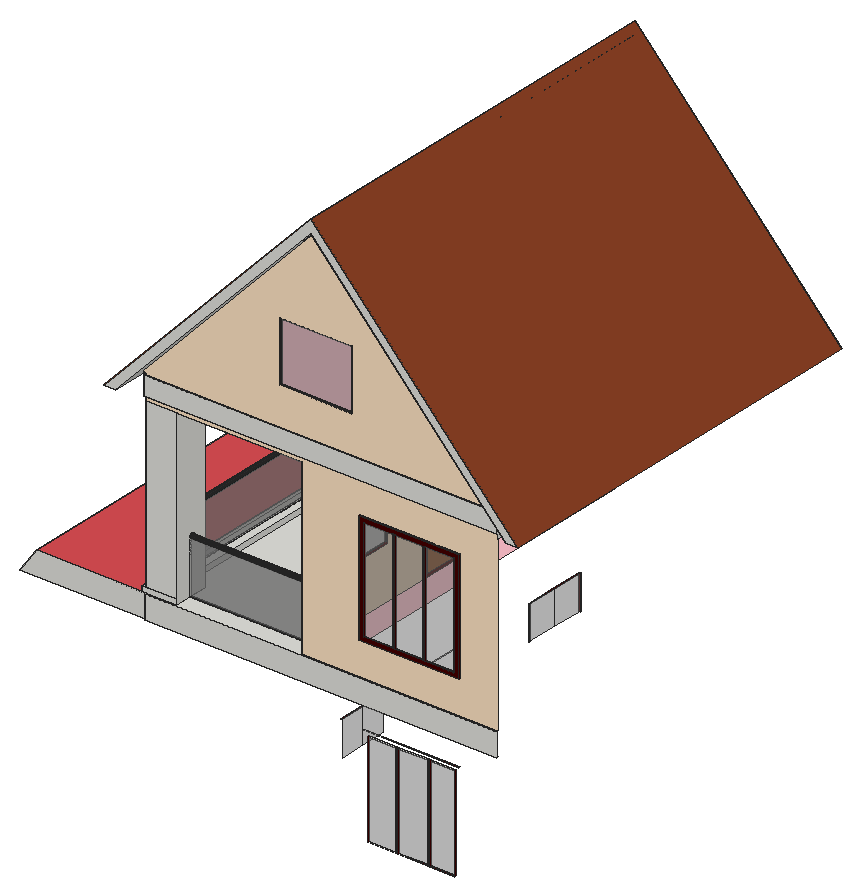
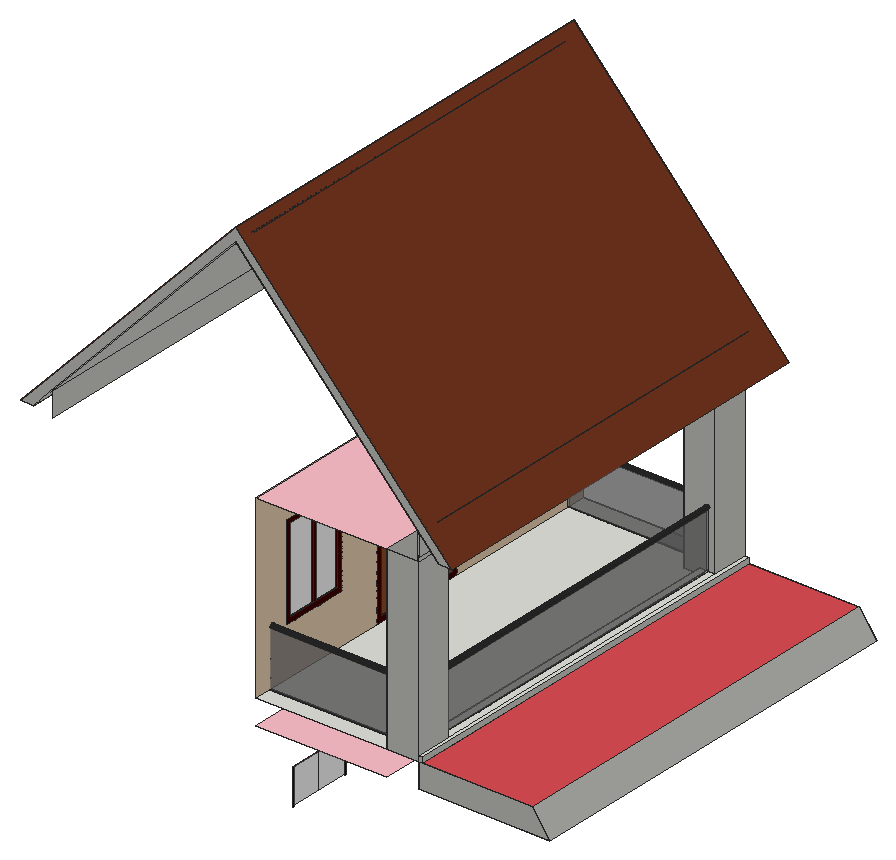
# SketchUp Ruby script. Lengths in inches.
U = 1.inch
M = Sketchup.active_model
def pt(a) = Geom::Point3d.new(a.map { |v| v * U })
def face(e, loops, mat)
  f = e.add_face(loops[0].map { |a| pt(a) })
  loops[1..].each { |l| e.add_face(l.map { |a| pt(a) }).erase! }
  f.material = f.back_material = mat if mat
  f
end
# faces: each face lists its corners as indices into pts; further lists are holes
def faces(e, pts, list, mat = nil) = list.each { |f| face(e, (f[0].is_a?(Array) ? f : [f]).map { |l| l.map { |i| pts[i] } }, mat) }
# xy, xz, yz: faces in a plane at the given z, y or x. An outline is a flat list of corners, or four numbers for a rectangle; further outlines are holes
def ring(l) = l.size == 4 ? [[l[0], l[1]], [l[2], l[1]], [l[2], l[3]], [l[0], l[3]]] : l.each_slice(2).to_a
def flat(e, list, mat, &to3) = list.each { |f| face(e, (f[0].is_a?(Array) ? f : [f]).map { |l| ring(l).map { |u, v| to3.(u, v) } }, mat) }
def xy(e, z, list, mat = nil) = flat(e, list, mat) { |x, y| [x, y, z] }
def xz(e, y, list, mat = nil) = flat(e, list, mat) { |x, z| [x, y, z] }
def yz(e, x, list, mat = nil) = flat(e, list, mat) { |y, z| [x, y, z] }
def lines(e, pts, list) = list.each { |a, b| e.add_line(pt(pts[a]), pt(pts[b])) }
# prism: a flat outline (further loops are holes) pulled along v
def prism(e, loops, v, mat = nil)
  f = face(e, loops, mat); d = Geom::Vector3d.new(v.map { |x| x * U })
  f.pushpull(f.normal.samedirection?(d) ? d.length : -d.length)
end
def box(e, o, s, mat = nil) = prism(e, [[o, [o[0] + s[0], o[1], o[2]], [o[0] + s[0], o[1] + s[1], o[2]], [o[0], o[1] + s[1], o[2]]]], [0, 0, s[2]], mat)
def at(x, y, z, deg = 0) = Geom::Transformation.translation(pt([x, y, z])) * Geom::Transformation.rotation(ORIGIN, Z_AXIS, deg.degrees)
def axes(o, x, y, z) = Geom::Transformation.new([*x, 0, *y, 0, *z, 0, *pt(o).to_a, 1])
def part(name) = M.definitions.add(name)
# library, detail: a bought-in or finely detailed component or shape, given as its bounding box
def library(name, o, s) = part(name).tap { |d| box(d.entities, o, s) }
def detail(e, o, s) = box(e.add_group.entities, o, s)
def put(e, d, t, mat = nil) = e.add_instance(d, t).tap { |i| i.material = mat if mat }
def group(e, t, mat = nil) = e.add_group.tap { |g| g.transformation = t; g.material = mat if mat }.entities
root = M.entities
M.materials.add("[0006_Pink]").color = [255, 192, 203]
M.materials.add("[0012_Bisque]").color = [255, 228, 196]
M.materials.add("[0022_Maroon]").color = [68, 0, 0]
M.materials.add("[0137_Black]").color = [45, 45, 45]
M.materials.add("[Roofing Scalloped Ornate]").color = [219, 78, 83]
M.materials.add("[Roofing Tile Spanish]").color = [138, 64, 36]
M.materials.add("[Translucent Glass Gray]").color = [128, 128, 128]
M.materials["[Translucent Glass Gray]"].alpha = 0.5
M.materials.add("[Wood Cherry Original]").color = [152, 86, 42]
xy(root,126.66,[[577.0625,82,581.0625,84],[625.98,82,629.98,84]])
xy(root,126.66,[[535.0625,82,577.0625,84],[581.0625,82,625.98,84],[629.98,82,667.98,84]],"[0022_Maroon]")
xy(root,140.25,[[432,383.84,434,385.71],[432,397.59,434,399.46]])
xy(root,163.32,[[432,383.84,434,385.71],[432,397.59,434,399.46]])
xy(root,226.5,[[432,159.23,434,238.92],[432,518.52,434,566.6875],[432,566.6875,434,614.85]],"[0022_Maroon]")
xy(root,227.44,[[432,334.98,434,391.49],[432,391.49,434,447.99]])
xy(root,271.7,[[535.0625,82,577.0625,84],[577.0625,82,581.0625,84],[581.0625,82,625.98,84],[625.98,82,629.98,84],[629.98,82,667.98,84]])
xy(root,278.46,[[528.3,82,674.74,84]],"[0022_Maroon]")
xy(root,312,[[432,82,732,84]])
xy(root,312,[[193.3125,82,193.3125,84,240,84,240,138.5625,193.3125,138.5625,193.3125,629.4375,240,629.4375,240,684,432,684,432,82],[0,84,193.3125,684]],"[0006_Pink]")
xy(root,348,[[193.3125,82,432,82,432,109.28,240,109.28,240,84,193.3125,84],[432,82,732,84],[187.3125,84,193.3125,138.5625],[193.3125,84,240,138.5625],[240,109.28,432,111.28],
  [240,111.28,432,111.28,432,656.72,240,656.72,240,629.4375,216.66,629.4375,216.66,138.5625,240,138.5625],[187.3125,138.5625,193.3125,629.4375],[193.3125,138.5625,216.66,629.4375],[187.3125,629.4375,193.3125,684],[193.3125,629.4375,240,684],
  [240,656.72,432,658.72],[240,658.72,432,684]])
xy(root,348,[[25.13,84,187.3125,684]],"[Roofing Scalloped Ornate]")
xy(root,355.14,[[432,322.1875,434,389.08],[432,389.08,434,455.96]],"[0022_Maroon]")
xy(root,356,[[187.3125,84,193.3125,684],[193.3125,138.5625,202.98,629.4375],[202.98,138.5625,204.98,629.4375],[204.98,138.5625,216.66,629.4375]])
xy(root,399.1,[[521.24,82,673.49,84]])
xy(root,406.125,[[572.26,82,576.26,84],[618.46,82,622.46,84]])
xy(root,406.125,[[528.26,82,572.26,84],[576.26,82,618.46,84],[622.46,82,666.46,84]],"[0022_Maroon]")
xy(root,427.0625,[[432,534.59,434,574.62],[432,578.62,434,622.65]],"[0022_Maroon]")
xy(root,429,[[240,109.28,432,111.28],[240,656.72,432,658.72]])
xy(root,432.76,[[432,157.6,434,195.91],[432,199.91,434,242.21]],"[0022_Maroon]")
xy(root,437,[[202.98,138.5625,204.98,629.4375]])
xy(root,447.4,[[432,378.54,434,380.85],[432,395.92,434,398.23]])
xy(root,473.15,[[432,378.54,434,380.85],[432,395.92,434,398.23]])
xy(root,551.5,[[432,157.6,434,195.91],[432,199.91,434,242.21],[432,534.59,434,574.62],[432,578.62,434,622.65]],"[0022_Maroon]")
xy(root,551.61,[[432,389.08,434,455.96]])
xy(root,551.61,[[432,322.1875,434,389.08]],"[0022_Maroon]")
xy(root,563.02,[[572.26,82,576.26,84],[618.46,82,622.46,84]])
xy(root,563.02,[[528.26,82,572.26,84],[576.26,82,618.46,84],[622.46,82,666.46,84]],"[0022_Maroon]")
xy(root,570.04,[[521.24,82,673.49,84]],"[0022_Maroon]")
xy(root,612,[[240,84,240,138.5625,193.3125,138.5625,193.3125,629.4375,240,629.4375,240,684,432,684,432,84]],"[0006_Pink]")
xy(root,619.2,[[191.3125,82,732,84],[191.3125,84,193.3125,684]])
xy(root,621.68,[[141.01,68.125,160.14,688.3125],[756.56,68.125,775.69,688.3125]])
xy(root,648,[[191.3125,82,732,84],[191.3125,84,193.3125,684]])
xy(root,705.51,[[398.35,84,509.29,87]],"[0137_Black]")
xy(root,798.07,[[398.35,84,509.29,87]],"[0137_Black]")
xz(root,68.125,[[141.01,621.68,160.14,621.68,458.35,941.28,756.56,621.68,775.69,621.68,458.35,961.79]])
xz(root,82,[[193.3125,312,732,348],[191.3125,619.2,732,648]])
xz(root,82,[[577.0625,126.66,581.0625,271.7],[625.98,126.66,629.98,271.7],[[521.24,399.1,673.49,570.04],[528.26,406.125,666.46,563.02]],[572.26,406.125,576.26,563.02],[618.46,406.125,622.46,563.02]],"[0022_Maroon]")
xz(root,84,[[577.0625,126.66,581.0625,271.7],[625.98,126.66,629.98,271.7],[0,312,193.3125,312,193.3125,348,25.13,348],[187.3125,348,240,356],[193.3125,356,240,612],
  [[521.24,399.1,673.49,570.04],[528.26,406.125,666.46,563.02]],[572.26,406.125,576.26,563.02],[618.46,406.125,622.46,563.02]])
xz(root,84,[[[432,348,732,348,732,619.2,193.3125,619.2,193.3125,612,432,612],[521.24,399.1,673.49,570.04]],[[193.3125,648,732,648,462.66,936,457.75,940.59,188.41,652.59],[398.35,705.51,509.29,798.07]]],"[0012_Bisque]")
xz(root,84,[[535.0625,126.66,577.0625,271.7],[581.0625,126.66,625.98,271.7],[629.98,126.66,667.98,271.7],[528.26,406.125,572.26,563.02],[576.26,406.125,618.46,563.02],
  [622.46,406.125,666.46,563.02]],"[Translucent Glass Gray]")
xz(root,87,[[398.35,705.51,509.29,798.07]],"[Translucent Glass Gray]")
xz(root,109.28,[[240,348,432,429]],"[Translucent Glass Gray]")
xz(root,111.28,[[240,429,432,432]])
xz(root,111.28,[[240,348,432,429]],"[Translucent Glass Gray]")
xz(root,138.5625,[[[216.66,348,216.66,356,193.3125,356,193.3125,612,240,612,240,348],[204.98,437,205.76,437.1,206.48,437.4,207.11,437.88,207.58,438.5,207.88,439.22,207.98,440,207.88,440.78,207.58,441.5,207.11,442.12,206.48,442.6,205.76,442.9,204.98,443,204.21,442.9,203.48,442.6,202.86,442.12,202.39,441.5,202.09,440.78,201.98,440,202.09,439.22,202.39,438.5,202.86,437.88,203.48,437.4,204.21,437.1]],[202.98,356,204.98,437]])
xz(root,157.6,[[432,432.76,434,551.5]])
xz(root,195.91,[[432,432.76,434,551.5]],"[0022_Maroon]")
xz(root,199.91,[[432,432.76,434,551.5]],"[0022_Maroon]")
xz(root,242.21,[[432,432.76,434,551.5]],"[0022_Maroon]")
xz(root,322.1875,[[432,355.14,434,551.61]],"[0022_Maroon]")
xz(root,378.54,[[432,447.4,434,473.15]])
xz(root,380.85,[[432,447.4,434,473.15]])
xz(root,383.84,[[432,140.25,434,163.32]])
xz(root,385.71,[[432,140.25,434,163.32]])
xz(root,395.92,[[432,447.4,434,473.15]])
xz(root,397.59,[[432,140.25,434,163.32]])
xz(root,398.23,[[432,447.4,434,473.15]])
xz(root,399.46,[[432,140.25,434,163.32]])
xz(root,455.96,[[432,355.14,434,551.61]],"[0022_Maroon]")
xz(root,518.52,[[432,174.15,434,226.5]],"[0022_Maroon]")
xz(root,534.59,[[432,427.0625,434,551.5]],"[0022_Maroon]")
xz(root,574.62,[[432,427.0625,434,551.5]],"[0022_Maroon]")
xz(root,578.62,[[432,427.0625,434,551.5]],"[0022_Maroon]")
xz(root,614.85,[[432,174.15,434,226.5]],"[0022_Maroon]")
xz(root,622.65,[[432,427.0625,434,551.5]],"[0022_Maroon]")
xz(root,629.4375,[[[216.66,348,240,348,240,612,193.3125,612,193.3125,356,216.66,356],[204.98,437,204.21,437.1,203.48,437.4,202.86,437.88,202.39,438.5,202.09,439.22,201.98,440,202.09,440.78,202.39,441.5,202.86,442.12,203.48,442.6,204.21,442.9,204.98,443,205.76,442.9,206.48,442.6,207.11,442.12,207.58,441.5,207.88,440.78,207.98,440,207.88,439.22,207.58,438.5,207.11,437.88,206.48,437.4,205.76,437.1]],[202.98,356,204.98,437],[204.98,437,204.21,437.1,203.48,437.4,202.86,437.88,202.39,438.5,202.09,439.22,201.98,440,202.09,440.78,202.39,441.5,202.86,442.12,203.48,442.6,204.21,442.9,204.98,443,205.76,442.9,206.48,442.6,207.11,442.12,207.58,441.5,207.88,440.78,207.98,440,207.88,439.22,207.58,438.5,207.11,437.88,206.48,437.4,205.76,437.1]])
xz(root,656.72,[[240,429,432,432]])
xz(root,656.72,[[240,348,432,429]],"[Translucent Glass Gray]")
xz(root,658.72,[[240,348,432,429]],"[Translucent Glass Gray]")
xz(root,684,[[0,312,25.13,348,193.3125,348,193.3125,312],[187.3125,348,193.3125,356],[193.3125,348,240,612]])
xz(root,688.3125,[[141.01,621.68,458.35,961.79,775.69,621.68,756.56,621.68,732,648,458.35,941.28,160.14,621.68]])
yz(root,187.3125,[[84,348,684,356]])
yz(root,191.3125,[[82,619.2,684,648]])
yz(root,193.3125,[[82,312,84,348],[84,312,684,348],[84,356,138.5625,612],[629.4375,356,684,612],[84,612,684,619.2]])
yz(root,202.98,[[138.5625,356,629.4375,437]],"[Translucent Glass Gray]")
yz(root,204.98,[[138.5625,437,629.4375,440]])
yz(root,204.98,[[138.5625,356,629.4375,437]],"[Translucent Glass Gray]")
yz(root,216.66,[[138.5625,348,629.4375,356]])
yz(root,240,[[84,348,109.28,348,109.28,429,111.28,429,110.5,429.1,109.78,429.4,109.16,429.88,108.68,430.5,108.38,431.22,108.28,432,108.38,432.78,108.68,433.5,109.16,434.12,109.78,434.6,110.5,434.9,111.28,435,112.06,434.9,112.78,434.6,113.4,434.12,113.88,433.5,114.18,432.78,114.28,432,114.18,431.22,113.88,430.5,113.4,429.88,112.78,429.4,112.06,429.1,111.28,429,111.28,348,138.5625,348,138.5625,612,84,612],[109.28,348,111.28,429],[[629.4375,348,684,612],[656.72,429,655.94,429.1,655.22,429.4,654.6,429.88,654.12,430.5,653.82,431.22,653.72,432,653.82,432.78,654.12,433.5,654.6,434.12,655.22,434.6,655.94,434.9,656.72,435,657.5,434.9,658.22,434.6,658.84,434.12,659.32,433.5,659.62,432.78,659.72,432,659.62,431.22,659.32,430.5,658.84,429.88,658.22,429.4,657.5,429.1]],[656.72,348,658.72,429],[111.28,429,110.5,429.1,109.78,429.4,109.16,429.88,108.68,430.5,108.38,431.22,108.28,432,108.38,432.78,108.68,433.5,109.16,434.12,109.78,434.6,110.5,434.9,111.28,435,112.06,434.9,112.78,434.6,113.4,434.12,113.88,433.5,114.18,432.78,114.28,432,114.18,431.22,113.88,430.5,113.4,429.88,112.78,429.4,112.06,429.1],
  [656.72,429,655.94,429.1,655.22,429.4,654.6,429.88,654.12,430.5,653.82,431.22,653.72,432,653.82,432.78,654.12,433.5,654.6,434.12,655.22,434.6,655.94,434.9,656.72,435,657.5,434.9,658.22,434.6,658.84,434.12,659.32,433.5,659.62,432.78,659.72,432,659.62,431.22,659.32,430.5,658.84,429.88,658.22,429.4,657.5,429.1]])
yz(root,398.35,[[84,705.51,87,798.07]],"[0137_Black]")
yz(root,432,[[383.84,140.25,385.71,163.32],[397.59,140.25,399.46,163.32],[109.28,348,111.28,429],[656.72,348,658.72,429],[378.54,447.4,380.85,473.15],
  [395.92,447.4,398.23,473.15]])
yz(root,432,[[[84,348,84,612,684,612,684,348,463.11,348,463.11,558.75,315.04,558.75,315.04,348],[527.34,419.8125,629.9,558.75],[152.78,427.94,247.03,556.32],[111.28,429,112.06,429.1,112.78,429.4,113.4,429.88,113.88,430.5,114.18,431.22,114.28,432,114.18,432.78,113.88,433.5,113.4,434.12,112.78,434.6,112.06,434.9,111.28,435,110.5,434.9,109.78,434.6,109.16,434.12,108.68,433.5,108.38,432.78,108.28,432,108.38,431.22,108.68,430.5,109.16,429.88,109.78,429.4,110.5,429.1],[656.72,429,657.5,429.1,658.22,429.4,658.84,429.88,659.32,430.5,659.62,431.22,659.72,432,659.62,432.78,659.32,433.5,658.84,434.12,658.22,434.6,657.5,434.9,656.72,435,655.94,434.9,655.22,434.6,654.6,434.12,654.12,433.5,653.82,432.78,653.72,432,653.82,431.22,654.12,430.5,654.6,429.88,655.22,429.4,655.94,429.1]]],"[0012_Bisque]")
yz(root,432,[[[315.04,348,463.11,558.75],[322.1875,355.14,455.96,551.61]],[[527.34,419.8125,629.9,558.75],[534.59,427.0625,622.65,551.5]],[574.62,427.0625,578.62,551.5],[[152.78,427.94,247.03,556.32],[157.6,432.76,242.21,551.5]],[195.91,432.76,199.91,551.5]],"[0022_Maroon]")
yz(root,434,[[159.23,172.5,199.08,226.5],[199.08,172.5,238.92,226.5],[518.52,174.15,566.6875,226.5],[566.6875,174.15,614.85,226.5],[534.59,427.0625,574.62,551.5],
  [578.62,427.0625,622.65,551.5],[157.6,432.76,195.91,551.5],[199.91,432.76,242.21,551.5]],"[Translucent Glass Gray]")
yz(root,434,[[[322.1875,355.14,389.08,551.61],[378.54,447.4,380.85,473.15]],[[389.08,355.14,455.96,551.61],[395.92,447.4,398.23,473.15]]],"[Wood Cherry Original]")
yz(root,509.29,[[84,705.51,87,798.07]],"[0137_Black]")
yz(root,521.24,[[82,399.1,84,570.04]],"[0022_Maroon]")
yz(root,528.26,[[82,406.125,84,563.02]],"[0022_Maroon]")
yz(root,535.0625,[[82,126.66,84,271.7]],"[0022_Maroon]")
yz(root,572.26,[[82,406.125,84,563.02]],"[0022_Maroon]")
yz(root,576.26,[[82,406.125,84,563.02]],"[0022_Maroon]")
yz(root,577.0625,[[82,126.66,84,271.7]],"[0022_Maroon]")
yz(root,581.0625,[[82,126.66,84,271.7]],"[0022_Maroon]")
yz(root,618.46,[[82,406.125,84,563.02]],"[0022_Maroon]")
yz(root,622.46,[[82,406.125,84,563.02]],"[0022_Maroon]")
yz(root,625.98,[[82,126.66,84,271.7]],"[0022_Maroon]")
yz(root,629.98,[[82,126.66,84,271.7]],"[0022_Maroon]")
yz(root,666.46,[[82,406.125,84,563.02]],"[0022_Maroon]")
yz(root,667.98,[[82,126.66,84,271.7]],"[0022_Maroon]")
yz(root,673.49,[[82,399.1,84,570.04]],"[0022_Maroon]")
yz(root,732,[[84,612,684,612,684,648,82,648,82,619.2,84,619.2]])
p = [[25.13,84,348],[25.13,684,348],[0,684,312],[0,84,312],[240,110.5,429.1],[240,111.28,429],
  [432,111.28,429],[432,110.5,429.1],[240,112.06,429.1],[432,112.06,429.1],[240,655.94,429.1],[240,656.72,429],
  [432,656.72,429],[432,655.94,429.1],[240,657.5,429.1],[432,657.5,429.1],[240,109.78,429.4],[432,109.78,429.4],
  [240,112.78,429.4],[432,112.78,429.4],[240,655.22,429.4],[432,655.22,429.4],[240,658.22,429.4],[432,658.22,429.4],
  [240,109.16,429.88],[432,109.16,429.88],[240,113.4,429.88],[432,113.4,429.88],[240,654.6,429.88],[432,654.6,429.88],
  [240,658.84,429.88],[432,658.84,429.88],[240,108.68,430.5],[432,108.68,430.5],[240,113.88,430.5],[432,113.88,430.5],
  [240,654.12,430.5],[432,654.12,430.5],[240,659.32,430.5],[432,659.32,430.5],[240,108.38,431.22],[432,108.38,431.22],
  [240,114.18,431.22],[432,114.18,431.22],[240,653.82,431.22],[432,653.82,431.22],[240,659.62,431.22],[432,659.62,431.22],
  [240,108.28,432],[432,108.28,432],[240,114.28,432],[432,114.28,432],[240,653.72,432],[432,653.72,432],
  [240,659.72,432],[432,659.72,432],[240,108.38,432.78],[432,108.38,432.78],[240,114.18,432.78],[432,114.18,432.78],
  [240,653.82,432.78],[432,653.82,432.78],[240,659.62,432.78],[432,659.62,432.78],[240,108.68,433.5],[432,108.68,433.5],
  [240,113.88,433.5],[432,113.88,433.5],[240,654.12,433.5],[432,654.12,433.5],[240,659.32,433.5],[432,659.32,433.5],
  [240,109.16,434.12],[432,109.16,434.12],[240,113.4,434.12],[432,113.4,434.12],[240,654.6,434.12],[432,654.6,434.12],
  [240,658.84,434.12],[432,658.84,434.12],[240,109.78,434.6],[432,109.78,434.6],[240,112.78,434.6],[432,112.78,434.6],
  [240,655.22,434.6],[432,655.22,434.6],[240,658.22,434.6],[432,658.22,434.6],[240,110.5,434.9],[432,110.5,434.9],
  [240,112.06,434.9],[432,112.06,434.9],[240,655.94,434.9],[432,655.94,434.9],[240,657.5,434.9],[432,657.5,434.9],
  [240,111.28,435],[432,111.28,435],[240,656.72,435],[432,656.72,435],[204.21,629.4375,437.1],[204.98,629.4375,437],
  [204.98,138.5625,437],[204.21,138.5625,437.1],[205.76,629.4375,437.1],[205.76,138.5625,437.1],[203.48,629.4375,437.4],[203.48,138.5625,437.4],
  [206.48,629.4375,437.4],[206.48,138.5625,437.4],[202.86,629.4375,437.88],[202.86,138.5625,437.88],[207.11,629.4375,437.88],[207.11,138.5625,437.88],
  [202.39,629.4375,438.5],[202.39,138.5625,438.5],[207.58,629.4375,438.5],[207.58,138.5625,438.5],[202.09,629.4375,439.22],[202.09,138.5625,439.22],
  [207.88,629.4375,439.22],[207.88,138.5625,439.22],[201.98,629.4375,440],[201.98,138.5625,440],[207.98,629.4375,440],[207.98,138.5625,440],
  [202.09,629.4375,440.78],[202.09,138.5625,440.78],[207.88,629.4375,440.78],[207.88,138.5625,440.78],[202.39,629.4375,441.5],[202.39,138.5625,441.5],
  [207.58,629.4375,441.5],[207.58,138.5625,441.5],[202.86,629.4375,442.12],[202.86,138.5625,442.12],[207.11,629.4375,442.12],[207.11,138.5625,442.12],
  [203.48,629.4375,442.6],[203.48,138.5625,442.6],[206.48,629.4375,442.6],[206.48,138.5625,442.6],[204.21,629.4375,442.9],[204.21,138.5625,442.9],
  [205.76,629.4375,442.9],[205.76,138.5625,442.9],[204.98,629.4375,443],[204.98,138.5625,443],[141.01,68.125,621.68],[458.35,68.125,961.79],
  [458.35,688.3125,961.79],[141.01,688.3125,621.68],[458.35,68.125,941.28],[160.14,68.125,621.68],[160.14,688.3125,621.68],[458.35,688.3125,941.28],
  [756.56,68.125,621.68],[732,688.3125,648],[756.56,688.3125,621.68],[775.69,68.125,621.68],[775.69,688.3125,621.68],[193.3125,684,648],
  [193.3125,84,648],[188.41,84,652.59],[188.41,684,652.59],[462.66,84,936],[732,84,648],[732,684,648],
  [462.66,684,936],[457.75,84,940.59],[457.75,684,940.59]]
faces(root,p,[[0,1,2,3],[152,153,154,155],[156,152,155,157,158],[161,162,163,164],[165,166,167,168],[163,169,170,164],[165,168,170,169]])
faces(root,p,[[4,5,6,7],[5,8,9,6],[10,11,12,13],[11,14,15,12],[16,4,7,17],[8,18,19,9],[20,10,13,21],[14,22,23,15],
  [24,16,17,25],[18,26,27,19],[28,20,21,29],[22,30,31,23],[32,24,25,33],[26,34,35,27],[36,28,29,37],[30,38,39,31],
  [40,32,33,41],[34,42,43,35],[44,36,37,45],[38,46,47,39],[48,40,41,49],[42,50,51,43],[52,44,45,53],[46,54,55,47],
  [56,48,49,57],[50,58,59,51],[60,52,53,61],[54,62,63,55],[64,56,57,65],[58,66,67,59],[68,60,61,69],[62,70,71,63],
  [72,64,65,73],[66,74,75,67],[76,68,69,77],[70,78,79,71],[80,72,73,81],[74,82,83,75],[84,76,77,85],[78,86,87,79],
  [88,80,81,89],[82,90,91,83],[92,84,85,93],[86,94,95,87],[96,88,89,97],[90,96,97,91],[98,92,93,99],[94,98,99,95],
  [100,101,102,103],[101,104,105,102],[106,100,103,107],[104,108,109,105],[110,106,107,111],[108,112,113,109],[114,110,111,115],[112,116,117,113],
  [118,114,115,119],[116,120,121,117],[122,118,119,123],[120,124,125,121],[126,122,123,127],[124,128,129,125],[130,126,127,131],[128,132,133,129],
  [134,130,131,135],[132,136,137,133],[138,134,135,139],[136,140,141,137],[142,138,139,143],[140,144,145,141],[146,142,143,147],[144,146,147,145]],"[0137_Black]")
faces(root,p,[[148,149,150,151],[149,159,160,150]],"[Roofing Tile Spanish]")
lines(root,p,[[157,167]])
